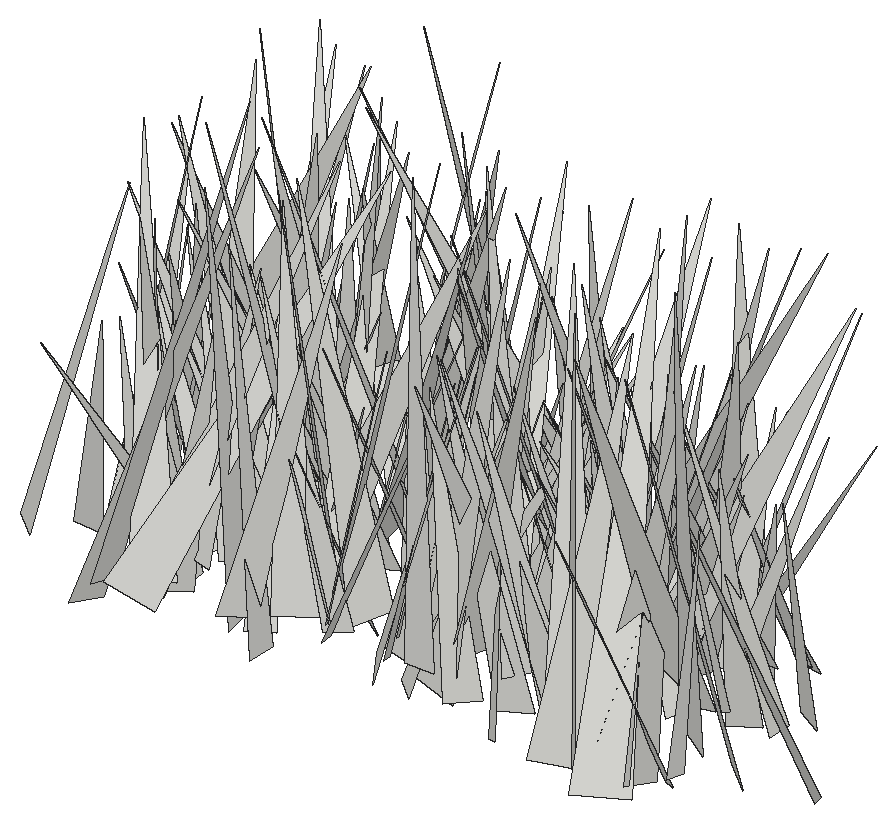
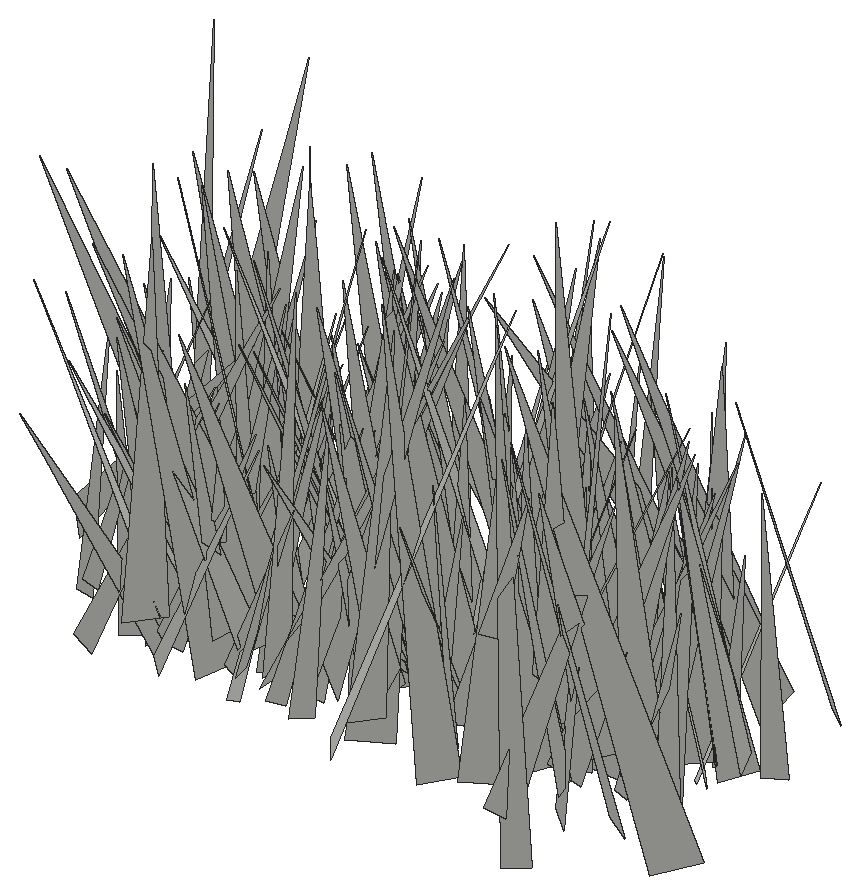
# SketchUp Ruby script. Lengths in inches.
U = 1.inch
M = Sketchup.active_model
def pt(a) = Geom::Point3d.new(a.map { |v| v * U })
def face(e, loops, mat)
  f = e.add_face(loops[0].map { |a| pt(a) })
  loops[1..].each { |l| e.add_face(l.map { |a| pt(a) }).erase! }
  f.material = f.back_material = mat if mat
  f
end
# faces: each face lists its corners as indices into pts; further lists are holes
def faces(e, pts, list, mat = nil) = list.each { |f| face(e, (f[0].is_a?(Array) ? f : [f]).map { |l| l.map { |i| pts[i] } }, mat) }
# xy, xz, yz: faces in a plane at the given z, y or x. An outline is a flat list of corners, or four numbers for a rectangle; further outlines are holes
def ring(l) = l.size == 4 ? [[l[0], l[1]], [l[2], l[1]], [l[2], l[3]], [l[0], l[3]]] : l.each_slice(2).to_a
def flat(e, list, mat, &to3) = list.each { |f| face(e, (f[0].is_a?(Array) ? f : [f]).map { |l| ring(l).map { |u, v| to3.(u, v) } }, mat) }
def xy(e, z, list, mat = nil) = flat(e, list, mat) { |x, y| [x, y, z] }
def xz(e, y, list, mat = nil) = flat(e, list, mat) { |x, z| [x, y, z] }
def yz(e, x, list, mat = nil) = flat(e, list, mat) { |y, z| [x, y, z] }
def lines(e, pts, list) = list.each { |a, b| e.add_line(pt(pts[a]), pt(pts[b])) }
# prism: a flat outline (further loops are holes) pulled along v
def prism(e, loops, v, mat = nil)
  f = face(e, loops, mat); d = Geom::Vector3d.new(v.map { |x| x * U })
  f.pushpull(f.normal.samedirection?(d) ? d.length : -d.length)
end
def box(e, o, s, mat = nil) = prism(e, [[o, [o[0] + s[0], o[1], o[2]], [o[0] + s[0], o[1] + s[1], o[2]], [o[0], o[1] + s[1], o[2]]]], [0, 0, s[2]], mat)
def at(x, y, z, deg = 0) = Geom::Transformation.translation(pt([x, y, z])) * Geom::Transformation.rotation(ORIGIN, Z_AXIS, deg.degrees)
def axes(o, x, y, z) = Geom::Transformation.new([*x, 0, *y, 0, *z, 0, *pt(o).to_a, 1])
def part(name) = M.definitions.add(name)
# library, detail: a bought-in or finely detailed component or shape, given as its bounding box
def library(name, o, s) = part(name).tap { |d| box(d.entities, o, s) }
def detail(e, o, s) = box(e.add_group.entities, o, s)
def put(e, d, t, mat = nil) = e.add_instance(d, t).tap { |i| i.material = mat if mat }
def group(e, t, mat = nil) = e.add_group.tap { |g| g.transformation = t; g.material = mat if mat }.entities
root = M.entities
c1 = part("fur_instance\#9")
p = [[0.8125,0,1.79],[0.67,-0.02,1.48],[0,-0.11,0],[0,0.11,0]]
faces(c1.entities,p,[[0,1,2,3]])
put(root,c1,axes([118.72,193.76,-28.22],[-6.68895,-1.28776,2.75903],[-1.15,7.23488,0.5888],[2.81923,-0.10417,6.78629]))
put(root,c1,axes([120.45,192.43,-28.22],[-5.92753,-0.80933,1.51712],[-1.07571,5.99367,-1.00549],[1.34146,1.2301,5.89742]))
put(root,c1,axes([131.3,192.92,-28.22],[4.46233,4.90899,2.88894],[5.22756,-4.98695,0.39938],[-2.26203,-1.84084,6.62202]))
put(root,c1,axes([133.07,196.11,-27.1],[1.39715,-7.46285,0.32526],[-7.45597,-1.41344,-0.40331],[-0.45656,0.24497,7.58179]))
put(root,c1,axes([134.2,193.77,-28.22],[-2.45002,-3.17903,0.27674],[-3.09062,2.27713,-1.20338],[-0.79426,0.94543,3.82893]))
put(root,c1,axes([116.26,193.7,-28.22],[3.71133,-3.4553,1.19556],[-3.62183,-3.7076,0.52772],[-0.50083,1.20708,5.04327]))
put(root,c1,axes([135.3,192.67,-27.1],[-3.53887,0.08812,1.47041],[-0.2173,3.75324,-0.74791],[1.45693,0.77383,3.46005]))
put(root,c1,axes([119.8125,192.14,-27.1],[-4.5359,3.17744,2.60533],[2.766,5.23085,-1.56386],[3.0386,-0.01843,5.3127]))
put(root,c1,axes([121.87,194.28,-27.1],[-4.72321,-4.87597,2.05821],[-5.0831,4.94763,0.05633],[1.47426,1.43735,6.78828]))
put(root,c1,axes([126.65,193.82,-28.22],[2.55776,-3.86723,2.22173],[-4.13899,-3.01226,-0.47827],[-1.66143,1.55064,4.61182]))
put(root,c1,axes([111.76,192.57,-27.1],[3.62165,4.35293,0.90177],[4.41878,-3.65214,-0.11732],[-0.48531,-0.76904,5.66132]))
put(root,c1,axes([121.12,193.16,-27.1],[-2.98056,5.41129,1.99239],[5.72855,3.03527,0.32601],[0.65987,-1.90801,6.16924]))
put(root,c1,axes([130.91,192.61,-28.22],[-3.21117,5.73542,2.2751],[5.803,3.67883,-1.08356],[2.09673,-1.39782,6.48325]))
put(root,c1,axes([130.49,193.96,-28.22],[-0.87207,-5.64239,2.10409],[-5.67136,0.05471,-2.20385],[-2.02471,2.277,5.26688]))
put(root,c1,axes([129.51,194.75,-28.22],[-5.01187,1.13995,1.85475],[1.60842,5.07616,1.22637],[1.46717,-1.67079,4.99142]))
put(root,c1,axes([123.49,193.79,-28.22],[5.2265,3.38981,1.10604],[3.55749,-5.09026,-1.20993],[-0.2416,-1.62138,6.11091]))
put(root,c1,axes([134.3125,194.625,-27.1],[3.79237,5.90894,3.79832],[6.9076,-3.92109,-0.79686],[-1.27587,-3.6653,6.97586]))
put(root,c1,axes([122.59,193.24,-27.1],[-0.71726,5.0627,1.58469],[5.02661,0.13746,1.836],[-1.69568,-1.73401,4.77227]))
put(root,c1,axes([125.57,193.82,-28.22],[1.63751,6.97927,2.94123],[7.53115,-1.18196,-1.38823],[0.80173,-3.15202,7.03309]))
put(root,c1,axes([116.52,192.19,-27.1],[2.2285,7.10603,0.93052],[7.02267,-1.97084,-1.76797],[1.42959,-1.39565,7.23438]))
put(root,c1,axes([116.18,193.12,-27.1],[2.91004,3.86675,2.0314],[3.84438,-3.42612,1.0144],[-2.0734,-0.92551,4.73192]))
put(root,c1,axes([126.39,194.48,-27.1],[6.40795,-1.734,1.03011],[-1.73088,-6.48917,-0.15614],[-1.03535,0.11648,6.63658]))
put(root,c1,axes([115.55,191.41,-27.1],[-6.44163,0.17845,3.84936],[-1.24896,6.99677,-2.4144],[3.64548,2.71245,5.9747]))
put(root,c1,axes([116.66,192.24,-27.1],[-2.09458,6.39775,0.76013],[6.40195,1.97698,1.00139],[-0.72385,-1.02792,6.657]))
put(root,c1,axes([128.67,192.61,-28.22],[1.83922,3.08635,0.93557],[2.6886,-2.06216,1.51739],[-1.78108,0.07419,3.25666]))
put(root,c1,axes([135.45,195.27,-28.22],[-4.39451,-5.32367,1.29551],[-5.40377,4.48556,0.10243],[0.905,0.93264,6.90237]))
put(root,c1,axes([122.02,193.95,-27.1],[-7.0839,-2.86843,1.00142],[-2.98784,7.03787,-0.97651],[0.55097,1.28563,7.57997]))
put(root,c1,axes([114.625,191.77,-28.22],[7.28027,0.47928,1.68125],[-0.05604,-7.13268,2.27604],[-1.74733,2.22571,6.93193]))
put(root,c1,axes([128.19,194.31,-28.22],[0.21554,-5.31829,2.18174],[-5.56977,-0.73327,-1.23719],[-1.42193,2.0661,5.17688]))
put(root,c1,axes([113.76,196.71,-28.22],[-3.67716,-3.23058,0.06887],[-2.92053,3.36739,2.02339],[1.38271,-1.47883,4.45691]))
put(root,c1,axes([116.6875,191.14,-27.1],[-2.61013,7.00123,1.33294],[6.01827,2.92557,-3.58165],[3.81765,0.17478,6.55758]))
put(root,c1,axes([127.1,196.44,-28.22],[2.94915,-5.28887,0.70098],[-5.06545,-3.02722,-1.5291],[-1.67475,-0.15728,5.85931]))
put(root,c1,axes([112.04,195.1,-28.22],[0.87128,-4.23502,0.75689],[-4.24446,-0.72019,0.85631],[0.702,0.90186,4.23807]))
put(root,c1,axes([121.98,195.58,-28.22],[-1.91573,-3.10975,0.18965],[-3.07242,1.92263,0.49017],[0.51647,-0.09744,3.61944]))
put(root,c1,axes([114.49,195.82,-28.22],[5.63565,-3.00774,1.4531],[-2.80235,-5.80815,-1.15361],[-1.81792,-0.37081,6.28301]))
put(root,c1,axes([131.94,193.88,-27.1],[5.79665,-1.91222,1.6292],[-2.17494,-5.87047,0.84811],[-1.25719,1.33905,6.04471]))
put(root,c1,axes([116.87,193.91,-27.1],[0.82444,4.69785,1.50621],[4.90559,-0.61872,-0.75536],[0.52313,-1.60174,4.70945]))
put(root,c1,axes([130.95,193.27,-27.1],[-5.28353,4.19242,1.51467],[4.2139,5.46353,-0.42331],[1.45386,-0.59977,6.73148]))
put(root,c1,axes([116.26,194.64,-28.22],[-3.7389,-0.44853,0.79303],[-0.43438,3.82202,0.11371],[0.80087,-0.02096,3.764]))
put(root,c1,axes([122.89,194.4,-27.1],[-6.49588,1.72746,1.45223],[1.82521,6.62397,0.28488],[1.32729,-0.65455,6.71561]))
put(root,c1,axes([123.73,194.7,-28.22],[0.68635,-5.64905,2.27441],[-5.90756,-0.06201,1.6287],[1.47832,2.3749,5.45254]))
put(root,c1,axes([124.64,192.9,-27.1],[3.32895,2.2471,0.95718],[1.81279,-3.35751,1.57751],[-1.63691,0.85163,3.69362]))
put(root,c1,axes([125.71,193.03,-27.1],[1.80048,6.74236,1.9451],[6.61582,-2.30046,1.85022],[-2.33959,-1.31645,6.72888]))
put(root,c1,axes([124.93,193.38,-28.22],[3.32598,3.77438,0.4675],[3.78797,-3.34308,0.04133],[-0.34022,-0.32329,5.03054]))
put(root,c1,axes([119.625,193.42,-28.22],[-3.18277,2.93848,0.48438],[2.88307,3.21784,-0.5768],[0.74643,0.10079,4.29324]))
put(root,c1,axes([122.62,192.68,-27.1],[4.4552,2.25801,0.37031],[2.04407,-4.29173,1.57715],[-1.02836,1.2518,4.7392]))
put(root,c1,axes([133.13,191.97,-28.22],[-6.0602,5.67803,0.65626],[5.53411,6.06799,-1.39639],[1.4298,0.57987,8.18634]))
put(root,c1,axes([132.38,192.68,-27.1],[4.78963,3.34115,0.62659],[3.09789,-4.73577,1.57225],[-1.39963,0.95165,5.62422]))
put(root,c1,axes([123.64,195.65,-27.1],[4.61843,1.91697,0.98697],[2.11588,-4.47821,-1.2031],[-0.41467,-1.49987,4.85358]))
put(root,c1,axes([117.01,194.92,-27.1],[-3.73085,2.02538,0.45172],[2.07172,3.68874,0.57157],[0.11914,-0.71871,4.20651]))
put(root,c1,axes([117.73,194.61,-27.1],[-1.66438,3.94539,0.96796],[4.04045,1.49913,0.83702],[-0.42169,-1.20819,4.19948]))
put(root,c1,axes([124.32,194.98,-28.22],[4.92372,-1.23429,0.65682],[-1.32256,-4.89156,0.72207],[-0.45359,0.86432,5.02445]))
put(root,c1,axes([120.79,195.38,-27.1],[3.65523,2.01923,0.98653],[2.16689,-3.66612,-0.52479],[-0.59594,-0.94526,4.14277]))
put(root,c1,axes([121.82,193.94,-27.1],[6.24718,3.3719,1.68528],[3.2403,-6.4703,0.93425],[-1.92623,0.05148,7.03734]))
put(root,c1,axes([113.55,195.61,-28.22],[0.6335,-3.36408,1.34348],[-3.58683,-0.77327,-0.24494],[-0.50657,1.2682,3.41444]))
put(root,c1,axes([114.52,197.32,-27.1],[-1.82022,-4.66244,0.24993],[-4.60062,1.83672,0.75812],[0.79693,-0.04591,4.9474]))
put(root,c1,axes([130.55,197.54,-28.22],[-3.83157,-3.11067,0.41222],[-2.87249,3.73899,1.51524],[1.26294,-0.9332,4.69694]))
put(root,c1,axes([130.1875,196,-27.1],[-4.58656,-0.99691,0.53395],[-0.9871,4.61746,0.14195],[0.55187,-0.02624,4.69151]))
put(root,c1,axes([119.61,196.36,-27.1],[3.62629,-0.3933,0.08931],[-0.3696,-3.56406,-0.68808],[-0.16141,-0.67481,3.58206]))
put(root,c1,axes([133.125,195.57,-27.1],[-3.66432,1.46778,0.50332],[1.5223,3.65057,0.437],[0.30055,-0.59495,3.9231]))
put(root,c1,axes([122.01,198.16,-28.22],[-2.61623,-5.06997,0.16776],[-4.93297,2.58676,1.24576],[1.18261,-0.42604,5.56752]))
put(root,c1,axes([131.15,196.78,-27.1],[1.6386,-6.2759,2.07036],[-6.47654,-1.94928,-0.78297],[-1.31443,1.78093,6.43885]))
put(root,c1,axes([120.26,195.75,-28.22],[-3.73959,3.61146,1.09906],[3.77498,3.58144,1.07604],[0.00944,-1.53809,5.08619]))
put(root,c1,axes([133.54,193.26,-28.22],[-7.99125,0.08509,2.25297],[-0.74491,7.73167,-2.93422],[2.12796,3.02611,7.43355]))
put(root,c1,axes([119.24,195.74,-28.22],[1.82991,-7.19945,3.13467],[-7.38413,-0.48301,3.20126],[2.67073,3.59742,6.70317]))
put(root,c1,axes([125.04,195.52,-27.1],[3.37481,3.69249,0.11879],[3.55193,-3.19874,-1.47981],[1.01606,-1.08238,4.77849]))
put(root,c1,axes([121.48,196.94,-27.1],[-0.67131,-4.1889,0.93111],[-4.10147,0.34927,-1.38579],[-1.26165,1.09345,4.00962]))
put(root,c1,axes([130.76,198.69,-28.22],[-2.89154,-5.8907,0.51675],[-5.81601,2.937,0.93617],[1.06836,0.04534,6.49499]))
put(root,c1,axes([138.06,195.66,-28.22],[-4.35257,-4.39527,0.35538],[-3.69396,3.36161,-3.66659],[-2.40819,2.78761,4.98191]))
put(root,c1,axes([125.84,199.79,-28.22],[-3.49524,-7.20934,0.56433],[-6.86604,3.50524,2.25399],[2.26947,-0.49846,7.68835]))
put(root,c1,axes([119.22,198.02,-27.1],[-4.05728,-2.523,0.42943],[-2.40041,4.03064,1.00168],[0.88766,-0.63233,4.67158]))
put(root,c1,axes([128.2,194.55,-27.1],[-7.28792,0.99409,0.70676],[0.80322,7.1337,-1.75122],[0.9179,1.65037,7.1439]))
put(root,c1,axes([121.63,198.62,-27.1],[-5.81753,-5.50464,0.89808],[-5.45533,5.88597,0.73893],[1.16061,0.07452,7.97488]))
put(root,c1,axes([115.32,197.11,-28.22],[5.71322,-0.96407,0.62556],[-0.92485,-5.73993,-0.39936],[-0.68221,-0.29224,5.7802]))
put(root,c1,axes([119.02,198.68,-28.22],[6.25935,-4.83068,2.00086],[-4.50057,-6.56633,-1.77386],[-2.66155,-0.25726,7.70509]))
put(root,c1,axes([124.1,194.0625,-27.1],[3.59429,3.23742,0.8797],[2.57384,-3.488,2.32011],[-2.15177,1.23558,4.24464]))
put(root,c1,axes([117.62,197.43,-27.1],[4.3427,-1.50818,1.19732],[-1.3579,-4.49272,-0.73402],[-1.36538,-0.32877,4.53816]))
put(root,c1,axes([129.38,197.07,-28.22],[-4.9951,-5.23204,0.99068],[-5.30492,4.77148,-1.54841],[-0.46216,1.77916,7.06595]))
put(root,c1,axes([116.46,197.26,-27.1],[-5.398,0.07669,0.31538],[0.11355,5.36878,0.63804],[0.30406,-0.64352,5.36071]))
put(root,c1,axes([120.31,198.26,-27.1],[7.393,0.04175,0.28729],[0.1077,-7.1937,-1.72622],[-0.26959,-1.72907,7.18877]))
put(root,c1,axes([133.77,197.7,-28.22],[2.34766,-4.1804,1.05082],[-4.25289,-2.44131,-0.21062],[-0.70205,0.80976,4.78987]))
put(root,c1,axes([128.58,198.13,-28.22],[1.30695,-5.86281,0.96642],[-5.89292,-1.15208,0.98022],[0.76158,1.14664,5.9262]))
put(root,c1,axes([135.98,196.53,-27.1],[-5.12979,-1.0122,0.11272],[-1.018,5.07872,-0.72273],[-0.03042,0.73083,5.17851]))
put(root,c1,axes([116.33,198.92,-27.1],[2.3597,-7.64104,0.82634],[-7.58316,-2.17409,1.55097],[1.25061,1.23463,7.84527]))
put(root,c1,axes([113.58,196.47,-28.22],[3.13745,2.7412,0.96065],[2.81213,-3.22064,0.00574],[-0.7273,-0.62763,4.16626]))
put(root,c1,axes([112.97,195.66,-28.22],[-4.2045,3.84796,1.64776],[3.68267,4.51063,-1.13666],[1.98995,-0.21727,5.58504]))
put(root,c1,axes([130.92,198.84,-28.22],[-4.78281,-0.5343,0.54387],[-0.29464,4.48183,1.81189],[0.70318,-1.75621,4.45846]))
put(root,c1,axes([112.96,196.78,-27.1],[3.09566,2.75124,1.27433],[2.88928,-3.22895,-0.04754],[-0.91941,-0.88367,4.14127]))
put(root,c1,axes([112.03,196.5,-27.1],[5.547,2.87669,1.51326],[2.93945,-5.71712,0.09337],[-1.38744,-0.61131,6.24786]))
put(root,c1,axes([126.76,197.3,-27.1],[-0.37702,3.57753,2.02822],[3.88687,0.97529,-0.99777],[1.34335,-1.81786,3.4562]))
put(root,c1,axes([116.7,197.6,-28.22],[6.44965,-0.53992,1.19924],[-0.48241,-6.55498,-0.35669],[-1.22351,-0.26161,6.46237]))
put(root,c1,axes([124.21,197.77,-28.22],[4.00541,-4.88826,1.49079],[-5.10449,-3.91872,0.86522],[-0.24835,1.7057,6.26017]))
put(root,c1,axes([115.03,198.67,-28.22],[-1.78915,-3.44674,0.35763],[-3.41457,1.82215,0.479],[0.59044,0.09337,3.85378]))
put(root,c1,axes([134.09,196.47,-27.1],[-3.59352,-1.36236,0.30323],[-1.35819,3.22059,-1.62619],[-0.32136,1.6227,3.48208]))
put(root,c1,axes([112.78,199.51,-28.22],[4.81338,-2.70132,0.36004],[-2.51999,-4.69011,-1.49931],[-1.0375,-1.14068,5.31205]))
put(root,c1,axes([127.36,197.8,-27.1],[-2.83398,-2.56318,0.53676],[-2.6174,2.79801,-0.45803],[0.08496,0.70049,3.79362]))
put(root,c1,axes([130.67,198.18,-27.1],[3.4493,-3.36014,0.02886],[-3.29462,-3.37365,0.97621],[0.66096,0.719,4.71542]))
put(root,c1,axes([118.83,199.18,-28.22],[-5.82237,-2.50943,0.01956],[-2.48564,5.77362,0.82736],[0.34528,-0.75212,6.28591]))
put(root,c1,axes([124,197.0625,-28.22],[3.35941,2.47012,0.56366],[2.52325,-3.34641,-0.37364],[-0.22894,-0.63632,4.15301]))
put(root,c1,axes([116.94,198.375,-28.22],[1.42662,-4.11071,0.89066],[-4.20545,-1.41051,0.22612],[-0.07357,0.91596,4.34535]))
put(root,c1,axes([128.57,199.2,-27.1],[5.40312,-1.02873,0.51523],[-0.87968,-5.28821,-1.33359],[-0.74156,-1.2223,5.33606]))
put(root,c1,axes([126.33,195.79,-27.1],[-5.21181,1.32812,1.31914],[0.83689,5.14396,-1.87252],[1.67442,1.56295,5.04188]))
put(root,c1,axes([121.09,194.77,-27.1],[-5.92228,3.52878,0.304],[3.26745,5.67188,-2.1844],[1.36692,1.73077,6.53866]))
put(root,c1,axes([121.84,197.86,-28.22],[-0.91503,4.79321,2.31879],[5.31141,0.98733,0.05504],[0.37492,-2.28894,4.87946]))
put(root,c1,axes([122.79,200.83,-28.22],[6.38764,-4.10189,0.26345],[-3.90919,-6.21298,-1.95294],[-1.27011,-1.50671,7.33577]))
put(root,c1,axes([125.08,197.24,-27.1],[6.15209,3.35933,0.33959],[3.37614,-6.1107,-0.71393],[0.04606,-0.78923,6.97306]))
put(root,c1,axes([114.89,196.43,-28.22],[4.04294,1.47662,0.10602],[1.40514,-3.92456,1.07725],[-0.46609,0.97696,4.16717]))
put(root,c1,axes([124.16,197.29,-28.22],[3.25743,4.86298,0.41292],[4.6269,-2.91916,-2.12138],[1.55271,-1.50328,5.4552]))
put(root,c1,axes([133.24,199.375,-27.1],[-1.88046,-5.21634,0.33238],[-5.10911,1.75978,-1.28722],[-1.10347,0.74146,5.39346]))
put(root,c1,axes([124.36,199.13,-28.22],[1.67883,-4.20753,0.33675],[-4.18563,-1.61266,0.71764],[0.54516,0.57551,4.47289]))
put(root,c1,axes([128.65,197.85,-27.1],[5.36031,4.39922,1.5205],[4.6383,-5.24227,-1.18439],[-0.38885,-1.88772,6.83252]))
put(root,c1,axes([126.47,199.05,-28.22],[-6.87538,0.87455,0.95023],[1.06547,6.75006,1.49673],[0.72976,-1.61573,6.76724]))
put(root,c1,axes([130.35,198.34,-27.1],[-5.09295,0.86723,1.4086],[1.03106,5.23004,0.50795],[1.29351,-0.75432,5.14123]))
put(root,c1,axes([116.82,198.03,-28.22],[4.62251,0.92588,0.22465],[0.9419,-4.60847,-0.38752],[-0.14333,-0.42437,4.69837]))
put(root,c1,axes([116.32,198.01,-28.22],[0.94645,-5.69848,3.07489],[-6.04954,-1.88624,-1.63358],[-2.30884,2.60631,5.54074]))
put(root,c1,axes([131.15,199.84,-28.22],[6.44633,-3.37101,0.63256],[-3.2949,-6.46051,-0.8512],[-0.95262,-0.46602,7.22457]))
put(root,c1,axes([119.21,197.64,-28.22],[3.62939,6.32437,2.66269],[6.74766,-3.83695,-0.08396],[-1.24771,-2.35377,7.2913]))
put(root,c1,axes([121.52,195.63,-27.1],[6.37842,4.90538,1.53696],[4.59516,-6.53882,1.79932],[-2.30422,0.53885,7.84279]))
put(root,c1,axes([135.01,199.09,-28.22],[-1.38247,-3.90181,0.99129],[-3.91317,1.54858,0.63797],[0.94545,0.70412,4.09003]))
put(root,c1,axes([127.52,201.42,-28.22],[-3.26721,-5.06008,0.08616],[-4.54982,2.98181,2.58736],[2.21606,-1.33826,5.43917]))
put(root,c1,axes([126.4375,195.65,-27.1],[-1.83957,6.80237,0.25254],[6.80704,1.83779,0.08208],[-0.01336,-0.2652,7.04624]))
put(root,c1,axes([112.64,199.4375,-27.1],[-0.50328,-4.91347,1.0032],[-4.85841,0.72759,1.12622],[1.24277,0.85458,4.80907]))
put(root,c1,axes([130.57,198.54,-28.22],[3.23817,-2.36152,0.30304],[-2.37388,-3.16317,0.7165],[0.18248,0.75624,3.94324]))
put(root,c1,axes([127.75,199.36,-28.22],[3.30583,-2.31707,0.74955],[-2.21165,-3.38553,-0.71128],[-1.01942,-0.16893,3.97384]))
put(root,c1,axes([130.21,197.6,-28.22],[2.77972,-6.83526,2.99642],[-7.05556,-1.36449,3.4327],[2.43278,3.85274,6.53179]))
put(root,c1,axes([120.26,199.29,-27.1],[6.42408,-3.63909,0.41323],[-3.66082,-6.40525,0.50369],[-0.11006,0.64215,7.36601]))
put(root,c1,axes([125.6,196.95,-28.22],[3.6487,6.36792,1.23917],[6.47764,-3.65398,-0.29593],[-0.35515,-1.22351,7.3332]))
put(root,c1,axes([123.97,197.9,-27.1],[2.98745,4.37857,0.43851],[4.21633,-2.69647,-1.80015],[1.25963,-1.35874,4.98559]))
put(root,c1,axes([133,198.19,-27.1],[2.35379,3.88662,0.95748],[3.9563,-2.09005,-1.24191],[0.60851,-1.44527,4.3708]))
put(root,c1,axes([124.41,198.33,-27.1],[4.29417,-2.87763,1.75823],[-3.19183,-4.38696,0.6155],[-1.08829,1.5119,5.13243]))
put(root,c1,axes([127.4,197.92,-28.22],[2.40724,3.27999,1.19788],[3.2967,-2.61439,0.53362],[-1.15108,-0.62824,4.03341]))
put(root,c1,axes([114.85,197.83,-28.22],[-4.26519,0.30143,0.24037],[0.24291,4.17451,-0.92459],[0.29939,0.9072,4.17466]))
put(root,c1,axes([124.15,199.23,-27.1],[-6.04607,-3.24149,2.31572],[-3.3744,6.40425,0.15438],[2.11738,0.95032,6.85845]))
put(root,c1,axes([125.6,201.01,-27.1],[1.43774,-5.64122,0.58152],[-5.34924,-1.54822,-1.79367],[-1.88339,0.09091,5.53834]))
put(root,c1,axes([121.04,199.23,-28.22],[3.22787,2.03353,0.24614],[1.96333,-2.94045,-1.45397],[0.58408,-1.35405,3.52709]))
put(root,c1,axes([133.97,200.13,-27.1],[-1.2303,-3.6424,0.32202],[-3.65502,1.23499,0.00478],[0.10759,0.30356,3.84457]))
put(root,c1,axes([126.67,198.8,-28.22],[2.68991,-2.47286,1.2383],[-2.72716,-2.65872,0.6147],[-0.45937,1.30393,3.60178]))
put(root,c1,axes([132.68,198.53,-27.1],[-2.57998,2.99071,1.64125],[3.02202,2.95835,-0.64026],[1.58287,-0.77341,3.89753]))
put(root,c1,axes([126.14,201.31,-27.1],[-8.04638,-2.10125,0.20494],[-2.02323,7.90531,1.61682],[0.60315,-1.51404,8.15753]))
put(root,c1,axes([127.17,201.46,-27.1],[-6.19203,-3.31038,1.54754],[-2.85802,6.28451,2.00782],[2.2771,-1.114,6.72819]))
put(root,c1,axes([132.34,200.17,-28.22],[1.50872,-3.69838,0.31644],[-3.67115,-1.43625,0.71715],[0.54852,0.55997,3.92937]))
put(root,c1,axes([115.82,200.36,-27.1],[-0.4063,-5.76079,1.26429],[-5.69006,0.04941,-1.60344],[-1.5519,1.32705,5.54804]))
put(root,c1,axes([116.51,200.32,-27.1],[6.83641,-1.96558,0.32372],[-1.94381,-6.83529,-0.45298],[-0.43579,-0.34652,7.09893]))
put(root,c1,axes([117.53,199.88,-27.1],[1.49528,-4.80686,1.53266],[-5.04418,-1.45777,0.34917],[-0.10564,1.56838,5.02194]))
put(root,c1,axes([130.01,197.32,-27.1],[6.47636,2.00005,0.90058],[1.74291,-6.39683,1.67254],[-1.33173,1.35459,6.56857]))
put(root,c1,axes([127.65,199.71,-27.1],[-4.79801,0.15244,1.14259],[0.25589,4.91001,0.4195],[1.12396,-0.46714,4.78206]))
put(root,c1,axes([128.04,198.84,-27.1],[7.15691,-3.14413,0.26361],[-3.09126,-6.8566,2.14652],[0.63178,2.06831,7.5166]))
put(root,c1,axes([113.94,198.89,-27.1],[3.27303,-4.65782,3.06275],[-5.40234,-3.52629,0.41046],[-1.37496,2.76738,5.67799]))
put(root,c1,axes([124.3125,197.41,-28.22],[-0.90144,4.87523,0.09791],[4.65666,0.89022,-1.45364],[1.44671,0.1723,4.73998]))
put(root,c1,axes([122.52,198.06,-28.22],[5.6278,2.51424,1.57514],[2.22036,-5.80941,1.3399],[-1.96786,0.63554,6.01649]))
put(root,c1,axes([129.66,199.68,-28.22],[-0.77592,-4.15559,2.31409],[-4.39268,1.52537,1.26634],[1.82437,1.90534,4.03328]))
put(root,c1,axes([115.5,200.98,-28.22],[-5.15951,-5.90719,2.53837],[-5.9684,5.61072,0.92562],[2.3909,1.25844,7.78837]))
put(root,c1,axes([130.34,198.7,-27.1],[-3.13044,2.30171,0.23571],[2.28042,3.13636,-0.34054],[0.39127,0.13578,3.8706]))
put(root,c1,axes([123.11,200.35,-27.1],[3.6641,-0.22277,0.06955],[-0.2117,-3.63329,-0.48425],[-0.09821,-0.47926,3.63879]))
put(root,c1,axes([131.12,199.99,-28.22],[-1.9475,3.70978,1.3462],[3.85912,1.47603,1.51527],[-0.82582,-1.85103,3.9063]))
put(root,c1,axes([117.4375,202.27,-27.1],[4.70982,-4.44224,0.12242],[-4.38661,-4.67586,-0.90827],[-0.71149,-0.57769,6.41023]))
put(root,c1,axes([133.16,201.5,-28.22],[-1.6318,-4.41068,0.10105],[-4.3461,1.58854,-0.8456],[-0.75876,0.38671,4.62621]))
put(root,c1,axes([125.21,202.3,-27.1],[3.98276,-1.20965,1.22676],[-0.42908,-3.68899,-2.24451],[-1.66855,-1.93873,3.5054]))
put(root,c1,axes([130.77,198.78,-27.1],[0.96645,3.75371,0.08435],[3.72936,-0.9496,-0.47076],[0.43512,-0.19848,3.84744]))
put(root,c1,axes([128.98,200.02,-27.1],[4.01363,-0.60213,1.19124],[-0.70216,-4.16285,0.26162],[-1.13516,0.446,4.0501]))
put(root,c1,axes([117.58,198.61,-28.22],[-4.53452,6.13099,1.20513],[6.2123,4.58336,0.05748],[0.66981,-1.00349,7.62546]))
put(root,c1,axes([121.47,199.67,-28.22],[-4.39525,1.44739,0.73649],[1.42922,4.45652,-0.22883],[0.77116,-0.01,4.62177]))
put(root,c1,axes([126.4,200.74,-27.1],[5.75232,0.0292,2.58276],[0.25276,-6.28131,-0.49192],[-2.57052,-0.55229,5.73133]))
put(root,c1,axes([122.47,201.43,-27.1],[5.42089,-2.3865,1.81758],[-2.19868,-5.71457,-0.94576],[-2.04078,-0.18248,5.84696]))
put(root,c1,axes([128.19,199.85,-27.1],[5.44846,0.74036,0.07595],[0.73692,-5.44519,0.21553],[-0.10422,0.20337,5.4943]))
put(root,c1,axes([131.22,198.54,-27.1],[4.24517,2.47398,0.29086],[2.34061,-4.15824,1.20716],[-0.85248,0.90284,4.76286]))
put(root,c1,axes([124.87,200.18,-27.1],[-5.12266,-6.1706,2.10185],[-6.50165,4.64284,-2.21548],[-0.47189,3.01719,7.70776]))
put(root,c1,axes([128.49,200.2,-28.22],[0.00954,3.59248,1.3323],[3.47361,-0.5704,1.51319],[-1.6171,-1.20405,3.25826]))
put(root,c1,axes([130.64,201.18,-28.22],[-2.91318,-3.12111,0.33199],[-3.12229,2.8354,-0.74159],[-0.32068,0.74655,4.20452]))
put(root,c1,axes([129.01,200.27,-28.22],[6.46627,-2.11143,1.67342],[-2.36842,-6.52888,0.91405],[-1.28416,1.40953,6.74057]))
put(root,c1,axes([110.92,201.18,-28.22],[3.50419,-7.42751,1.71848],[-7.22357,-2.63012,3.36199],[2.43745,2.88357,7.49295]))
put(root,c1,axes([122.875,199.76,-27.1],[5.08359,-0.28901,1.82683],[-0.68576,-5.25683,1.07667],[-1.71772,1.24337,4.97667]))
put(root,c1,axes([131.36,200.8,-27.1],[4.8811,-3.48072,2.77846],[-3.79933,-5.40519,-0.09683],[-2.32386,1.52607,5.99426]))
put(root,c1,axes([131.47,199.88,-27.1],[4.74716,3.3592,0.52437],[3.38285,-4.75689,-0.1518],[-0.33985,-0.42721,5.81349]))
put(root,c1,axes([119.93,199.89,-27.1],[-3.53792,4.34861,0.23075],[4.30519,3.44804,1.02808],[-0.65501,-0.82532,5.51093]))
put(root,c1,axes([127.45,198.83,-27.1],[-1.69129,6.09931,0.73665],[6.01995,1.79783,-1.06428],[1.22654,-0.41345,6.23934]))
put(root,c1,axes([124.03,202.54,-27.1],[4.34393,-1.36952,0.92271],[-1.07858,-4.31928,-1.3331],[-1.25046,-1.03195,4.35524]))
put(root,c1,axes([119.15,201.43,-27.1],[3.83115,1.46002,1.29175],[1.69697,-3.89964,-0.62537],[-0.95945,-1.06731,4.05194]))
put(root,c1,axes([115.32,200.96,-27.1],[5.01565,1.80166,1.23073],[1.89818,-5.12441,-0.23415],[-1.07592,-0.64182,5.32428]))
put(root,c1,axes([122.2,203.46,-27.1],[-5.96811,-4.81477,0.42538],[-4.75156,5.96808,0.88657],[0.88638,-0.42578,7.61672]))
put(root,c1,axes([131.22,200.06,-28.22],[4.38555,-0.36882,0.03632],[-0.36139,-4.16033,1.38975],[0.08213,1.3878,4.17584]))
put(root,c1,axes([115.61,198.73,-27.1],[-4.47188,4.60163,0.40246],[4.4512,4.44255,-1.33612],[1.23441,0.65071,6.27595]))
put(root,c1,axes([114.6875,204.07,-28.22],[-1.84089,-7.99139,1.4242],[-7.16502,2.28604,3.56596],[3.81486,0.4373,7.3848]))
put(root,c1,axes([120.68,198.99,-27.1],[2.07794,4.44656,0.23399],[4.16362,-2.03187,1.63715],[-1.57826,0.49406,4.62704]))
put(root,c1,axes([118.5,202.95,-27.1],[6.88515,-2.28469,0.18682],[-2.24647,-6.84269,-0.88939],[-0.45618,-0.78602,7.19959]))
put(root,c1,axes([113.86,200.32,-28.22],[3.861,5.57007,1.34937],[5.71182,-3.87341,-0.35436],[-0.47072,-1.31331,6.76812]))
put(root,c1,axes([115.79,203.46,-27.1],[0.74185,-5.118,0.35857],[-5.01336,-0.80012,-1.04825],[-1.09027,0.19676,5.06413]))
